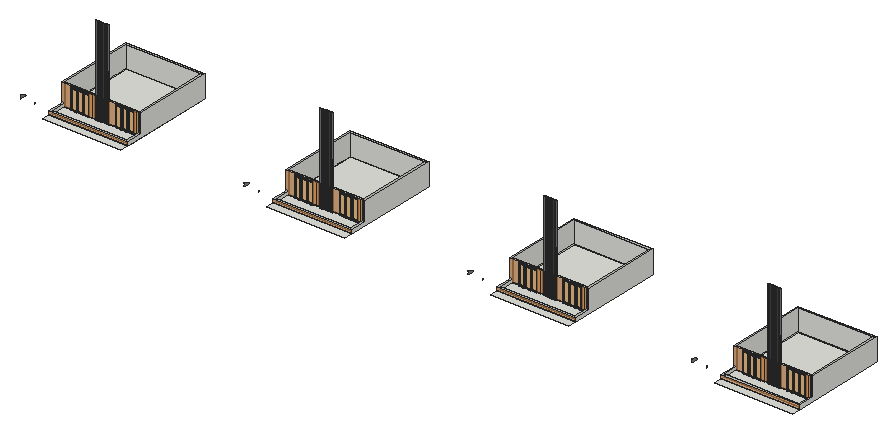
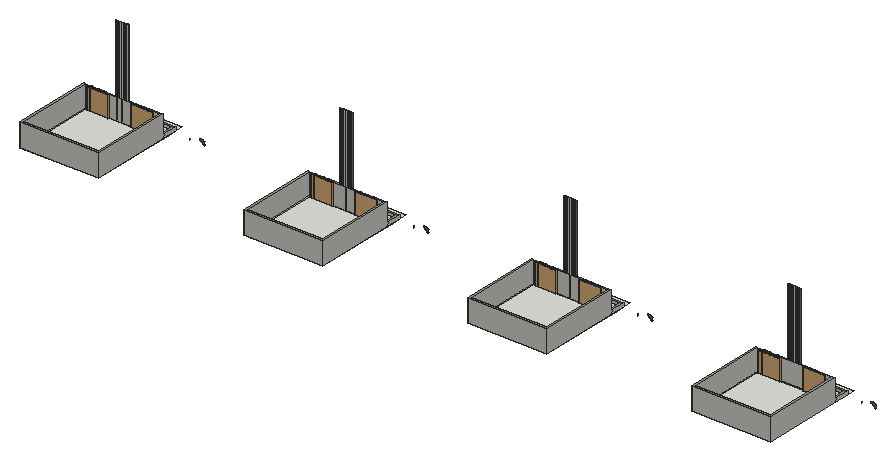
# SketchUp Ruby script. Lengths in inches.
U = 1.inch
M = Sketchup.active_model
def pt(a) = Geom::Point3d.new(a.map { |v| v * U })
def face(e, loops, mat)
  f = e.add_face(loops[0].map { |a| pt(a) })
  loops[1..].each { |l| e.add_face(l.map { |a| pt(a) }).erase! }
  f.material = f.back_material = mat if mat
  f
end
# faces: each face lists its corners as indices into pts; further lists are holes
def faces(e, pts, list, mat = nil) = list.each { |f| face(e, (f[0].is_a?(Array) ? f : [f]).map { |l| l.map { |i| pts[i] } }, mat) }
# xy, xz, yz: faces in a plane at the given z, y or x. An outline is a flat list of corners, or four numbers for a rectangle; further outlines are holes
def ring(l) = l.size == 4 ? [[l[0], l[1]], [l[2], l[1]], [l[2], l[3]], [l[0], l[3]]] : l.each_slice(2).to_a
def flat(e, list, mat, &to3) = list.each { |f| face(e, (f[0].is_a?(Array) ? f : [f]).map { |l| ring(l).map { |u, v| to3.(u, v) } }, mat) }
def xy(e, z, list, mat = nil) = flat(e, list, mat) { |x, y| [x, y, z] }
def xz(e, y, list, mat = nil) = flat(e, list, mat) { |x, z| [x, y, z] }
def yz(e, x, list, mat = nil) = flat(e, list, mat) { |y, z| [x, y, z] }
def lines(e, pts, list) = list.each { |a, b| e.add_line(pt(pts[a]), pt(pts[b])) }
# prism: a flat outline (further loops are holes) pulled along v
def prism(e, loops, v, mat = nil)
  f = face(e, loops, mat); d = Geom::Vector3d.new(v.map { |x| x * U })
  f.pushpull(f.normal.samedirection?(d) ? d.length : -d.length)
end
def box(e, o, s, mat = nil) = prism(e, [[o, [o[0] + s[0], o[1], o[2]], [o[0] + s[0], o[1] + s[1], o[2]], [o[0], o[1] + s[1], o[2]]]], [0, 0, s[2]], mat)
def at(x, y, z, deg = 0) = Geom::Transformation.translation(pt([x, y, z])) * Geom::Transformation.rotation(ORIGIN, Z_AXIS, deg.degrees)
def axes(o, x, y, z) = Geom::Transformation.new([*x, 0, *y, 0, *z, 0, *pt(o).to_a, 1])
def part(name) = M.definitions.add(name)
# library, detail: a bought-in or finely detailed component or shape, given as its bounding box
def library(name, o, s) = part(name).tap { |d| box(d.entities, o, s) }
def detail(e, o, s) = box(e.add_group.entities, o, s)
def put(e, d, t, mat = nil) = e.add_instance(d, t).tap { |i| i.material = mat if mat }
def group(e, t, mat = nil) = e.add_group.tap { |g| g.transformation = t; g.material = mat if mat }.entities
root = M.entities
M.materials.add("Wine2").color = [0, 0, 0]
M.materials["Wine2"].alpha = 0
M.materials.add("[0043_SaddleBrown]4").color = [124, 123, 122]
M.materials.add("[0130_Gainsboro]").color = [39, 45, 50]
M.materials.add("[Granite Dark Gray]").color = [69, 68, 68]
M.materials.add("[Stone Vein Gray]").color = [119, 119, 119]
M.materials.add("[Wood Floor]").color = [224, 152, 88]
M.materials["[Wood Floor]"].alpha = 0.68
c1 = part("Framed glazing panel")
xy(c1.entities,0,[[0,-0.98,43.07,0],[0,0,43.07,1.4]],"[0130_Gainsboro]")
xy(c1.entities,0.3,[[0.3,-1.43,42.77,-0.98]],"[0130_Gainsboro]")
xy(c1.entities,2.95,[[2.95,-1.43,40.12,-0.63],[2.95,-0.63,40.12,0],[2.95,0,40.12,0.64],[2.95,0.64,40.12,1.4]],"[0130_Gainsboro]")
xy(c1.entities,3.54,[[3.54,-0.63,39.53,0],[3.54,0,39.53,0.64]],"[0130_Gainsboro]")
xy(c1.entities,111.8125,[[3.54,-0.63,39.53,0],[3.54,0,39.53,0.64]],"[0130_Gainsboro]")
xy(c1.entities,112.4,[[2.95,-1.43,40.12,-0.63],[2.95,-0.63,40.12,0],[2.95,0,40.12,0.64],[2.95,0.64,40.12,1.4]],"[0130_Gainsboro]")
xy(c1.entities,115.05,[[0.3,-1.43,42.77,-0.98]],"[0130_Gainsboro]")
xy(c1.entities,115.35,[[0,-0.98,43.07,0],[0,0,43.07,1.4]],"[0130_Gainsboro]")
xz(c1.entities,-1.43,[[[0.3,0.3,42.77,115.05],[2.95,2.95,40.12,112.4]]],"[0130_Gainsboro]")
xz(c1.entities,-0.98,[[[0,0,43.07,115.35],[0.3,0.3,42.77,115.05]]],"[0130_Gainsboro]")
xz(c1.entities,-0.63,[[[2.95,2.95,40.12,112.4],[3.54,3.54,39.53,111.8125]]],"[0130_Gainsboro]")
xz(c1.entities,0,[[3.54,3.54,39.53,111.8125]],"Wine2")
xz(c1.entities,0,[[[0,0,43.07,115.35],[2.95,2.95,40.12,112.4]],[[2.95,2.95,40.12,112.4],[3.54,3.54,39.53,111.8125]]],"[0130_Gainsboro]")
xz(c1.entities,0.64,[[[2.95,2.95,40.12,112.4],[3.54,3.54,39.53,111.8125]]],"[0130_Gainsboro]")
xz(c1.entities,1.4,[[[0,0,43.07,115.35],[2.95,2.95,40.12,112.4]]],"[0130_Gainsboro]")
yz(c1.entities,0,[[-0.98,0,0,115.35],[0,0,1.4,115.35]],"[0130_Gainsboro]")
yz(c1.entities,0.3,[[-1.43,0.3,-0.98,115.05]],"[0130_Gainsboro]")
yz(c1.entities,2.95,[[-1.43,2.95,-0.63,112.4],[-0.63,2.95,0,112.4],[0,2.95,0.64,112.4],[0.64,2.95,1.4,112.4]],"[0130_Gainsboro]")
yz(c1.entities,3.54,[[-0.63,3.54,0,111.8125],[0,3.54,0.64,111.8125]],"[0130_Gainsboro]")
yz(c1.entities,39.53,[[-0.63,3.54,0,111.8125],[0,3.54,0.64,111.8125]],"[0130_Gainsboro]")
yz(c1.entities,40.12,[[-1.43,2.95,-0.63,112.4],[-0.63,2.95,0,112.4],[0,2.95,0.64,112.4],[0.64,2.95,1.4,112.4]],"[0130_Gainsboro]")
yz(c1.entities,42.77,[[-1.43,0.3,-0.98,115.05]],"[0130_Gainsboro]")
yz(c1.entities,43.07,[[-0.98,0,0,115.35],[0,0,1.4,115.35]],"[0130_Gainsboro]")
c2 = part("Glazing assembly")
put(c2.entities,c1,axes([90.57,1.43,0],[1.05148,0,0],[0,1,0],[0,0,1]))
put(c2.entities,c1,axes([0,1.43,0],[1.05148,0,0],[0,1,0],[0,0,1]))
put(c2.entities,c1,axes([45.29,1.43,0],[1.05148,0,0],[0,1,0],[0,0,1]))
c3 = library("Curtains",[0,0,0],[121.73,8.19,117.22])
xy(root,268.25,[[563.08,657.03,978.86,1085.17],[1813.71,657.03,2229.49,1085.17],[3064.33,657.03,3480.11,1085.17],[4314.96,657.03,4730.74,1085.17]])
xy(root,268.4375,[[551.76,515.0625,990.19,559.875],[1802.38,515.0625,2240.81,559.875],[3053.01,515.0625,3491.44,559.875],[4303.63,515.0625,4742.06,559.875],[551.76,559.875,990.19,589.17],
  [1802.38,559.875,2240.81,589.17],[3053.01,559.875,3491.44,589.17],[4303.63,559.875,4742.06,589.17],[[551.76,589.17,990.19,1096.5],[835.39,595.44,979.42,595.44,979.42,1090.24,558.02,1090.24,558.02,616,835.39,616]],[[1802.38,589.17,2240.81,1096.5],[2086.01,595.44,2230.05,595.44,2230.05,1090.24,1808.65,1090.24,1808.65,616,2086.01,616]],
  [[3053.01,589.17,3491.44,1096.5],[3336.64,595.44,3480.67,595.44,3480.67,1090.24,3059.27,1090.24,3059.27,616,3336.64,616]],[[4303.63,589.17,4742.06,1096.5],[4587.26,595.44,4731.3,595.44,4731.3,1090.24,4309.9,1090.24,4309.9,616,4587.26,616]]])
xy(root,274.4375,[[563.08,571.2,978.86,571.2,978.86,651.03,951.01,651.03,951.01,657.03,849.76,657.03,849.76,651.03,814.68,651.03,814.68,648.85,805.57,648.85,805.57,651.03,801.81,651.03,801.81,648.85,792.69,648.85,792.69,651.03,789.43,651.03,789.43,648.85,780.32,648.85,780.32,651.03,777.31,651.03,777.31,648.85,768.19,648.85,768.19,651.03,764.56,651.03,764.56,647.91,755.44,647.91,755.44,651.03,751.56,651.03,751.56,647.91,742.44,647.91,742.44,651.03,703.26,651.03,703.26,657.03,602.01,657.03,602.01,651.03,563.08,651.03],[1813.71,571.2,2229.49,571.2,2229.49,651.03,2201.63,651.03,2201.63,657.03,2100.38,657.03,2100.38,651.03,2065.31,651.03,2065.31,648.85,2056.19,648.85,2056.19,651.03,2052.43,651.03,2052.43,648.85,2043.32,648.85,2043.32,651.03,2040.06,651.03,2040.06,648.85,2030.94,648.85,2030.94,651.03,2027.93,651.03,2027.93,648.85,2018.82,648.85,2018.82,651.03,2015.18,651.03,2015.18,647.91,2006.07,647.91,2006.07,651.03,2002.18,651.03,2002.18,647.91,1993.07,647.91,1993.07,651.03,1953.89,651.03,1953.89,657.03,1852.64,657.03,1852.64,651.03,1813.71,651.03],[3064.33,571.2,3480.11,571.2,3480.11,651.03,3452.26,651.03,3452.26,657.03,3351.01,657.03,3351.01,651.03,3315.93,651.03,3315.93,648.85,3306.82,648.85,3306.82,651.03,3303.06,651.03,3303.06,648.85,3293.94,648.85,3293.94,651.03,3290.68,651.03,3290.68,648.85,3281.57,648.85,3281.57,651.03,3278.56,651.03,3278.56,648.85,3269.44,648.85,3269.44,651.03,3265.81,651.03,3265.81,647.91,3256.69,647.91,3256.69,651.03,3252.81,651.03,3252.81,647.91,3243.69,647.91,3243.69,651.03,3204.51,651.03,3204.51,657.03,3103.26,657.03,3103.26,651.03,3064.33,651.03],[4314.96,571.2,4730.74,571.2,4730.74,651.03,4702.88,651.03,4702.88,657.03,4601.63,657.03,4601.63,651.03,4566.56,651.03,4566.56,648.85,4557.44,648.85,4557.44,651.03,4553.68,651.03,4553.68,648.85,4544.57,648.85,4544.57,651.03,4541.31,651.03,4541.31,648.85,4532.19,648.85,4532.19,651.03,4529.18,651.03,4529.18,648.85,4520.07,648.85,4520.07,651.03,4516.43,651.03,4516.43,647.91,4507.32,647.91,4507.32,651.03,4503.43,651.03,4503.43,647.91,4494.32,647.91,4494.32,651.03,4455.14,651.03,4455.14,657.03,4353.89,657.03,4353.89,651.03,4314.96,651.03],[563.08,657.03,978.86,1085.17],
  [1813.71,657.03,2229.49,1085.17],[3064.33,657.03,3480.11,1085.17],[4314.96,657.03,4730.74,1085.17]])
xz(root,559.875,[[551.76,268.4375,990.19,289.5625],[1802.38,268.4375,2240.81,289.5625],[3053.01,268.4375,3491.44,289.5625],[4303.63,268.4375,4742.06,289.5625]],"[Wood Floor]")
xz(root,571.2,[[563.08,274.4375,978.86,289.5625],[1813.71,274.4375,2229.49,289.5625],[3064.33,274.4375,3480.11,289.5625],[4314.96,274.4375,4730.74,289.5625]])
xz(root,589.17,[[448.37,274.24,448.14,274.83,447.96,275.43,447.8125,276.04,447.71,276.65,447.65,277.26,447.625,277.875,447.65,278.49,447.71,279.11,447.8125,279.72,447.96,280.32,448.14,280.92,448.37,281.52],[1698.99,274.24,1698.77,274.83,1698.58,275.43,1698.4375,276.04,1698.33,276.65,1698.27,277.26,1698.25,277.875,1698.27,278.49,1698.33,279.11,1698.4375,279.72,1698.58,280.32,1698.77,280.92,1698.99,281.52],[2949.62,274.24,2949.39,274.83,2949.21,275.43,2949.0625,276.04,2948.96,276.65,2948.9,277.26,2948.875,277.875,2948.9,278.49,2948.96,279.11,2949.0625,279.72,2949.21,280.32,2949.39,280.92,2949.62,281.52],[4200.24,274.24,4200.02,274.83,4199.83,275.43,4199.6875,276.04,4199.58,276.65,4199.52,277.26,4199.5,277.875,4199.52,278.49,4199.58,279.11,4199.6875,279.72,4199.83,280.32,4200.02,280.92,4200.24,281.52],[367.98,274.88,367.98,278.09,368.99,279,369.85,279.99,370.53,281.06,371.02,282.17,371.32,283.32,371.42,284.48,371.32,285.65,371.02,286.8,370.53,287.91,369.85,288.98,368.99,289.97,367.98,290.875,367.98,291.93,369.26,292.12,370.53,292.36,371.79,292.65,373.02,292.98,374.22,293.37,375.39,293.79,376.54,294.26,377.64,294.77,378.71,295.33,379.74,295.92,380.72,296.55,381.65,297.22,382.38,297.73,383.16,298.2,383.98,298.63,384.84,299.02,385.74,299.36,386.67,299.65,387.625,299.9,388.6,300.09,389.6,300.24,390.61,300.33,391.62,300.37,392.64,300.36,393.45,300.26,394.22,300.04,394.89,299.69,395.4375,299.24,395.83,298.72,396.06,298.15,396.09,297.55,395.95,296.97,395.62,296.42,395.13,295.94,394.5,295.55,393.77,295.28,393.66,295.875,393.34,296.43,392.83,296.91,392.17,297.28,391.4,297.51,390.57,297.58,389.74,297.51,388.97,297.28,388.3,296.91,387.79,296.43,387.47,295.875,387.36,295.28,387.32,294.8,387.29,294.33,387.29,293.85,387.3,293.375,387.32,292.9,387.37,292.43,387.43,291.95,387.51,291.48,387.61,291.01,387.72,290.54,387.85,290.08,388,289.61,386.54,289.1875,385.13,288.68,383.78,288.1,382.49,287.43,381.29,286.7,380.17,285.9,379.14,285.04,378.2,284.12,377.375,283.15,376.66,282.14,376.05,281.09,375.57,280.01,375.04,279.51,374.5,279.02,373.93,278.54,373.34,278.07,372.73,277.625,372.11,277.1875,371.46,276.76,370.8,276.36,370.12,275.97,369.42,275.59,368.7,275.23],
  [1618.6,274.88,1618.6,278.09,1619.62,279,1620.48,279.99,1621.16,281.06,1621.65,282.17,1621.95,283.32,1622.05,284.48,1621.95,285.65,1621.65,286.8,1621.16,287.91,1620.48,288.98,1619.62,289.97,1618.6,290.875,1618.6,291.93,1619.89,292.12,1621.16,292.36,1622.41,292.65,1623.64,292.98,1624.85,293.37,1626.02,293.79,1627.16,294.26,1628.27,294.77,1629.33,295.33,1630.36,295.92,1631.34,296.55,1632.28,297.22,1633,297.73,1633.78,298.2,1634.6,298.63,1635.47,299.02,1636.36,299.36,1637.29,299.65,1638.25,299.9,1639.23,300.09,1640.23,300.24,1641.23,300.33,1642.25,300.37,1643.26,300.36,1644.08,300.26,1644.84,300.04,1645.52,299.69,1646.0625,299.24,1646.46,298.72,1646.68,298.15,1646.72,297.55,1646.57,296.97,1646.24,296.42,1645.75,295.94,1645.125,295.55,1644.39,295.28,1644.28,295.875,1643.96,296.43,1643.46,296.91,1642.79,297.28,1642.02,297.51,1641.19,297.58,1640.36,297.51,1639.59,297.28,1638.93,296.91,1638.42,296.43,1638.1,295.875,1637.99,295.28,1637.95,294.8,1637.92,294.33,1637.91,293.85,1637.92,293.375,1637.95,292.9,1637.99,292.43,1638.05,291.95,1638.13,291.48,1638.23,291.01,1638.35,290.54,1638.48,290.08,1638.63,289.61,1637.17,289.1875,1635.75,288.68,1634.4,288.1,1633.12,287.43,1631.91,286.7,1630.79,285.9,1629.76,285.04,1628.83,284.12,1628,283.15,1627.28,282.14,1626.68,281.09,1626.19,280.01,1625.67,279.51,1625.12,279.02,1624.55,278.54,1623.97,278.07,1623.36,277.625,1622.73,277.1875,1622.09,276.76,1621.42,276.36,1620.74,275.97,1620.04,275.59,1619.33,275.23],[2869.23,274.88,2869.23,278.09,2870.24,279,2871.1,279.99,2871.78,281.06,2872.27,282.17,2872.57,283.32,2872.67,284.48,2872.57,285.65,2872.27,286.8,2871.78,287.91,2871.1,288.98,2870.24,289.97,2869.23,290.875,2869.23,291.93,2870.51,292.12,2871.78,292.36,2873.04,292.65,2874.27,292.98,2875.47,293.37,2876.64,293.79,2877.79,294.26,2878.89,294.77,2879.96,295.33,2880.99,295.92,2881.97,296.55,2882.9,297.22,2883.63,297.73,2884.41,298.2,2885.23,298.63,2886.09,299.02,2886.99,299.36,2887.92,299.65,2888.875,299.9,2889.85,300.09,2890.85,300.24,2891.86,300.33,2892.87,300.37,2893.89,300.36,2894.7,300.26,2895.47,300.04,2896.14,299.69,2896.6875,299.24,2897.08,298.72,2897.31,298.15,2897.34,297.55,2897.2,296.97,2896.87,296.42,2896.38,295.94,2895.75,295.55,2895.02,295.28,2894.91,295.875,2894.59,296.43,2894.08,296.91,2893.42,297.28,2892.65,297.51,2891.82,297.58,2890.99,297.51,2890.22,297.28,2889.55,296.91,2889.04,296.43,2888.72,295.875,2888.61,295.28,2888.57,294.8,2888.54,294.33,2888.54,293.85,2888.55,293.375,2888.57,292.9,2888.62,292.43,2888.68,291.95,2888.76,291.48,2888.86,291.01,2888.97,290.54,2889.1,290.08,2889.25,289.61,2887.79,289.1875,2886.38,288.68,2885.03,288.1,2883.74,287.43,2882.54,286.7,2881.42,285.9,2880.39,285.04,2879.45,284.12,2878.625,283.15,2877.91,282.14,2877.3,281.09,2876.82,280.01,2876.29,279.51,2875.75,279.02,2875.18,278.54,2874.59,278.07,2873.98,277.625,2873.36,277.1875,2872.71,276.76,2872.05,276.36,2871.37,275.97,2870.67,275.59,2869.95,275.23],[4119.85,274.88,4119.85,278.09,4120.87,279,4121.73,279.99,4122.41,281.06,4122.9,282.17,4123.2,283.32,4123.3,284.48,4123.2,285.65,4122.9,286.8,4122.41,287.91,4121.73,288.98,4120.87,289.97,4119.85,290.875,4119.85,291.93,4121.14,292.12,4122.41,292.36,4123.66,292.65,4124.89,292.98,4126.1,293.37,4127.27,293.79,4128.41,294.26,4129.52,294.77,4130.58,295.33,4131.61,295.92,4132.59,296.55,4133.53,297.22,4134.25,297.73,4135.03,298.2,4135.85,298.63,4136.72,299.02,4137.61,299.36,4138.54,299.65,4139.5,299.9,4140.48,300.09,4141.48,300.24,4142.48,300.33,4143.5,300.37,4144.51,300.36,4145.33,300.26,4146.09,300.04,4146.77,299.69,4147.3125,299.24,4147.71,298.72,4147.93,298.15,4147.97,297.55,4147.82,296.97,4147.49,296.42,4147,295.94,4146.375,295.55,4145.64,295.28,4145.53,295.875,4145.21,296.43,4144.71,296.91,4144.04,297.28,4143.27,297.51,4142.44,297.58,4141.61,297.51,4140.84,297.28,4140.18,296.91,4139.67,296.43,4139.35,295.875,4139.24,295.28,4139.2,294.8,4139.17,294.33,4139.16,293.85,4139.17,293.375,4139.2,292.9,4139.24,292.43,4139.3,291.95,4139.38,291.48,4139.48,291.01,4139.6,290.54,4139.73,290.08,4139.88,289.61,4138.42,289.1875,4137,288.68,4135.65,288.1,4134.37,287.43,4133.16,286.7,4132.04,285.9,4131.01,285.04,4130.08,284.12,4129.25,283.15,4128.53,282.14,4127.93,281.09,4127.44,280.01,4126.92,279.51,4126.37,279.02,4125.8,278.54,4125.22,278.07,4124.61,277.625,4123.98,277.1875,4123.34,276.76,4122.67,276.36,4121.99,275.97,4121.29,275.59,4120.58,275.23]],"[0043_SaddleBrown]4")
xz(root,647.91,[[755.44,274.4375,764.56,771.4375],[2006.07,274.4375,2015.18,771.4375],[3256.69,274.4375,3265.81,771.4375],[4507.32,274.4375,4516.43,771.4375]],"[Granite Dark Gray]")
xz(root,647.91,[[742.44,274.4375,751.56,274.4375,751.56,771.4375,742.44,771.4375,742.44,665.9375,744.19,665.9375,744.19,662.4375,742.44,662.4375,742.44,541.1875,744.19,541.1875,744.19,538.1875,742.44,538.1875,742.44,413.5,744.38,413.5,744.38,410.625,742.44,410.625],[1993.07,274.4375,2002.18,274.4375,2002.18,771.4375,1993.07,771.4375,1993.07,665.9375,1994.82,665.9375,1994.82,662.4375,1993.07,662.4375,1993.07,541.1875,1994.82,541.1875,1994.82,538.1875,1993.07,538.1875,1993.07,413.5,1995.01,413.5,1995.01,410.625,1993.07,410.625],[3243.69,274.4375,3252.81,274.4375,3252.81,771.4375,3243.69,771.4375,3243.69,665.9375,3245.44,665.9375,3245.44,662.4375,3243.69,662.4375,3243.69,541.1875,3245.44,541.1875,3245.44,538.1875,3243.69,538.1875,3243.69,413.5,3245.63,413.5,3245.63,410.625,3243.69,410.625],[4494.32,274.4375,4503.43,274.4375,4503.43,771.4375,4494.32,771.4375,4494.32,665.9375,4496.07,665.9375,4496.07,662.4375,4494.32,662.4375,4494.32,541.1875,4496.07,541.1875,4496.07,538.1875,4494.32,538.1875,4494.32,413.5,4496.26,413.5,4496.26,410.625,4494.32,410.625]],"[Stone Vein Gray]")
xz(root,648.85,[[768.19,274.4375,777.31,771.4375],[780.32,274.4375,789.43,771.4375],[792.69,274.4375,801.81,771.4375],[2018.82,274.4375,2027.93,771.4375],[2030.94,274.4375,2040.06,771.4375],
  [2043.32,274.4375,2052.43,771.4375],[3269.44,274.4375,3278.56,771.4375],[3281.57,274.4375,3290.68,771.4375],[3293.94,274.4375,3303.06,771.4375],[4520.07,274.4375,4529.18,771.4375],
  [4532.19,274.4375,4541.31,771.4375],[4544.57,274.4375,4553.68,771.4375]],"[Granite Dark Gray]")
xz(root,648.85,[[805.57,274.4375,814.68,274.4375,814.68,662.4375,812.81,662.4375,812.81,665.9375,814.68,665.9375,814.68,771.4375,805.57,771.4375],[2056.19,274.4375,2065.31,274.4375,2065.31,662.4375,2063.43,662.4375,2063.43,665.9375,2065.31,665.9375,2065.31,771.4375,2056.19,771.4375],[3306.82,274.4375,3315.93,274.4375,3315.93,662.4375,3314.06,662.4375,3314.06,665.9375,3315.93,665.9375,3315.93,771.4375,3306.82,771.4375],[4557.44,274.4375,4566.56,274.4375,4566.56,662.4375,4564.68,662.4375,4564.68,665.9375,4566.56,665.9375,4566.56,771.4375,4557.44,771.4375]],"[Stone Vein Gray]")
xz(root,651.03,[[814.68,274.4375,814.89,410.625],[2065.31,274.4375,2065.52,410.625],[3315.93,274.4375,3316.14,410.625],[4566.56,274.4375,4566.77,410.625]])
xz(root,651.03,[[764.56,274.4375,768.19,771.4375],[777.31,274.4375,780.32,771.4375],[789.43,274.4375,792.69,771.4375],[2015.18,274.4375,2018.82,771.4375],[2027.93,274.4375,2030.94,771.4375],
  [2040.06,274.4375,2043.32,771.4375],[3265.81,274.4375,3269.44,771.4375],[3278.56,274.4375,3281.57,771.4375],[3290.68,274.4375,3293.94,771.4375],[4516.43,274.4375,4520.07,771.4375],
  [4529.18,274.4375,4532.19,771.4375],[4541.31,274.4375,4544.57,771.4375]],"[Granite Dark Gray]")
xz(root,651.03,[[751.56,274.4375,755.44,771.4375],[801.81,274.4375,805.57,771.4375],[2002.18,274.4375,2006.07,771.4375],[2052.43,274.4375,2056.19,771.4375],[3252.81,274.4375,3256.69,771.4375],
  [3303.06,274.4375,3306.82,771.4375],[4503.43,274.4375,4507.32,771.4375],[4553.68,274.4375,4557.44,771.4375]],"[Stone Vein Gray]")
xz(root,651.03,[[563.08,274.4375,602.01,274.4375,602.01,388.875,703.26,388.875,703.26,274.4375,742.44,274.4375,742.44,394.4375,551.76,394.4375,551.76,293,563.08,293],[814.89,274.4375,849.76,274.4375,849.76,388.875,951.01,388.875,951.01,274.4375,978.86,274.4375,978.86,394.4375,814.89,394.4375],[1813.71,274.4375,1852.64,274.4375,1852.64,388.875,1953.89,388.875,1953.89,274.4375,1993.07,274.4375,1993.07,394.4375,1802.38,394.4375,1802.38,293,1813.71,293],[2065.52,274.4375,2100.38,274.4375,2100.38,388.875,2201.63,388.875,2201.63,274.4375,2229.49,274.4375,2229.49,394.4375,2065.52,394.4375],[3064.33,274.4375,3103.26,274.4375,3103.26,388.875,3204.51,388.875,3204.51,274.4375,3243.69,274.4375,3243.69,394.4375,3053.01,394.4375,3053.01,293,3064.33,293],
  [3316.14,274.4375,3351.01,274.4375,3351.01,388.875,3452.26,388.875,3452.26,274.4375,3480.11,274.4375,3480.11,394.4375,3316.14,394.4375],[4314.96,274.4375,4353.89,274.4375,4353.89,388.875,4455.14,388.875,4455.14,274.4375,4494.32,274.4375,4494.32,394.4375,4303.63,394.4375,4303.63,293,4314.96,293],[4566.77,274.4375,4601.63,274.4375,4601.63,388.875,4702.88,388.875,4702.88,274.4375,4730.74,274.4375,4730.74,394.4375,4566.77,394.4375]],"[Wood Floor]")
xz(root,657.03,[[563.08,268.25,602.01,274.4375],[602.01,268.25,703.26,274.4375],[703.26,268.25,849.76,274.4375],[849.76,268.25,951.01,274.4375],[951.01,268.25,978.86,274.4375],
  [1813.71,268.25,1852.64,274.4375],[1852.64,268.25,1953.89,274.4375],[1953.89,268.25,2100.38,274.4375],[2100.38,268.25,2201.63,274.4375],[2201.63,268.25,2229.49,274.4375],
  [3064.33,268.25,3103.26,274.4375],[3103.26,268.25,3204.51,274.4375],[3204.51,268.25,3351.01,274.4375],[3351.01,268.25,3452.26,274.4375],[3452.26,268.25,3480.11,274.4375],
  [4314.96,268.25,4353.89,274.4375],[4353.89,268.25,4455.14,274.4375],[4455.14,268.25,4601.63,274.4375],[4601.63,268.25,4702.88,274.4375],[4702.88,268.25,4730.74,274.4375],
  [563.08,274.4375,563.08,394.4375,978.86,394.4375,978.86,274.4375,951.01,274.4375,951.01,388.875,849.76,388.875,849.76,274.4375,703.26,274.4375,703.26,388.875,602.01,388.875,602.01,274.4375],[1813.71,274.4375,1813.71,394.4375,2229.49,394.4375,2229.49,274.4375,2201.63,274.4375,2201.63,388.875,2100.38,388.875,2100.38,274.4375,1953.89,274.4375,1953.89,388.875,1852.64,388.875,1852.64,274.4375],[3064.33,274.4375,3064.33,394.4375,3480.11,394.4375,3480.11,274.4375,3452.26,274.4375,3452.26,388.875,3351.01,388.875,3351.01,274.4375,3204.51,274.4375,3204.51,388.875,3103.26,388.875,3103.26,274.4375],[4314.96,274.4375,4314.96,394.4375,4730.74,394.4375,4730.74,274.4375,4702.88,274.4375,4702.88,388.875,4601.63,388.875,4601.63,274.4375,4455.14,274.4375,4455.14,388.875,4353.89,388.875,4353.89,274.4375]])
xz(root,1085.17,[[563.08,268.25,978.86,274.4375],[1813.71,268.25,2229.49,274.4375],[3064.33,268.25,3480.11,274.4375],[4314.96,268.25,4730.74,274.4375],[563.08,274.4375,978.86,394.4375],
  [1813.71,274.4375,2229.49,394.4375],[3064.33,274.4375,3480.11,394.4375],[4314.96,274.4375,4730.74,394.4375]])
xz(root,1096.5,[[551.76,268.4375,990.19,394.4375],[1802.38,268.4375,2240.81,394.4375],[3053.01,268.4375,3491.44,394.4375],[4303.63,268.4375,4742.06,394.4375]])
yz(root,551.76,[[559.875,268.4375,640.11,289.5625],[640.11,268.4375,640.11,289.5625,651.03,289.5625,651.03,394.4375,1096.5,394.4375,1096.5,268.4375]])
yz(root,563.08,[[657.03,268.25,1085.17,274.4375],[571.2,274.4375,651.03,289.5625],[657.03,274.4375,1085.17,394.4375]])
yz(root,602.01,[[651.03,274.4375,657.03,388.875]])
yz(root,703.26,[[651.03,274.4375,657.03,388.875]])
yz(root,742.44,[[647.91,274.4375,651.03,394.4375]])
yz(root,751.56,[[647.91,274.4375,651.03,771.4375]])
yz(root,755.44,[[647.91,274.4375,651.03,394.4375]])
yz(root,764.56,[[647.91,274.4375,651.03,771.4375]])
yz(root,768.19,[[648.85,274.4375,651.03,394.4375]])
yz(root,777.31,[[648.85,274.4375,651.03,771.4375]])
yz(root,780.32,[[648.85,274.4375,651.03,394.4375]])
yz(root,789.43,[[648.85,274.4375,651.03,771.4375]])
yz(root,792.69,[[648.85,274.4375,651.03,394.4375]])
yz(root,801.81,[[648.85,274.4375,651.03,771.4375]])
yz(root,805.57,[[648.85,274.4375,651.03,394.4375]])
yz(root,814.68,[[648.85,274.4375,651.03,538.1875]])
yz(root,849.76,[[651.03,274.4375,657.03,388.875]])
yz(root,951.01,[[651.03,274.4375,657.03,388.875]])
yz(root,978.86,[[657.03,268.25,1085.17,274.4375],[571.2,274.4375,651.03,289.5625],[657.03,274.4375,1085.17,394.4375]])
yz(root,990.19,[[559.875,268.4375,1096.5,268.4375,1096.5,394.4375,651.03,394.4375,651.03,289.5625,559.875,289.5625]])
yz(root,1802.38,[[559.875,268.4375,640.11,289.5625],[640.11,268.4375,640.11,289.5625,651.03,289.5625,651.03,394.4375,1096.5,394.4375,1096.5,268.4375]])
yz(root,1813.71,[[657.03,268.25,1085.17,274.4375],[571.2,274.4375,651.03,289.5625],[657.03,274.4375,1085.17,394.4375]])
yz(root,1852.64,[[651.03,274.4375,657.03,388.875]])
yz(root,1953.89,[[651.03,274.4375,657.03,388.875]])
yz(root,1993.07,[[647.91,274.4375,651.03,394.4375]])
yz(root,2002.18,[[647.91,274.4375,651.03,771.4375]])
yz(root,2006.07,[[647.91,274.4375,651.03,394.4375]])
yz(root,2015.18,[[647.91,274.4375,651.03,771.4375]])
yz(root,2018.82,[[648.85,274.4375,651.03,394.4375]])
yz(root,2027.93,[[648.85,274.4375,651.03,771.4375]])
yz(root,2030.94,[[648.85,274.4375,651.03,394.4375]])
yz(root,2040.06,[[648.85,274.4375,651.03,771.4375]])
yz(root,2043.32,[[648.85,274.4375,651.03,394.4375]])
yz(root,2052.43,[[648.85,274.4375,651.03,771.4375]])
yz(root,2056.19,[[648.85,274.4375,651.03,394.4375]])
yz(root,2065.31,[[648.85,274.4375,651.03,538.1875]])
yz(root,2100.38,[[651.03,274.4375,657.03,388.875]])
yz(root,2201.63,[[651.03,274.4375,657.03,388.875]])
yz(root,2229.49,[[657.03,268.25,1085.17,274.4375],[571.2,274.4375,651.03,289.5625],[657.03,274.4375,1085.17,394.4375]])
yz(root,2240.81,[[559.875,268.4375,1096.5,268.4375,1096.5,394.4375,651.03,394.4375,651.03,289.5625,559.875,289.5625]])
yz(root,3053.01,[[559.875,268.4375,640.11,289.5625],[640.11,268.4375,640.11,289.5625,651.03,289.5625,651.03,394.4375,1096.5,394.4375,1096.5,268.4375]])
yz(root,3064.33,[[657.03,268.25,1085.17,274.4375],[571.2,274.4375,651.03,289.5625],[657.03,274.4375,1085.17,394.4375]])
yz(root,3103.26,[[651.03,274.4375,657.03,388.875]])
yz(root,3204.51,[[651.03,274.4375,657.03,388.875]])
yz(root,3243.69,[[647.91,274.4375,651.03,394.4375]])
yz(root,3252.81,[[647.91,274.4375,651.03,771.4375]])
yz(root,3256.69,[[647.91,274.4375,651.03,394.4375]])
yz(root,3265.81,[[647.91,274.4375,651.03,771.4375]])
yz(root,3269.44,[[648.85,274.4375,651.03,394.4375]])
yz(root,3278.56,[[648.85,274.4375,651.03,771.4375]])
yz(root,3281.57,[[648.85,274.4375,651.03,394.4375]])
yz(root,3290.68,[[648.85,274.4375,651.03,771.4375]])
yz(root,3293.94,[[648.85,274.4375,651.03,394.4375]])
yz(root,3303.06,[[648.85,274.4375,651.03,771.4375]])
yz(root,3306.82,[[648.85,274.4375,651.03,394.4375]])
yz(root,3315.93,[[648.85,274.4375,651.03,538.1875]])
yz(root,3351.01,[[651.03,274.4375,657.03,388.875]])
yz(root,3452.26,[[651.03,274.4375,657.03,388.875]])
yz(root,3480.11,[[657.03,268.25,1085.17,274.4375],[571.2,274.4375,651.03,289.5625],[657.03,274.4375,1085.17,394.4375]])
yz(root,3491.44,[[559.875,268.4375,1096.5,268.4375,1096.5,394.4375,651.03,394.4375,651.03,289.5625,559.875,289.5625]])
yz(root,4303.63,[[559.875,268.4375,640.11,289.5625],[640.11,268.4375,640.11,289.5625,651.03,289.5625,651.03,394.4375,1096.5,394.4375,1096.5,268.4375]])
yz(root,4314.96,[[657.03,268.25,1085.17,274.4375],[571.2,274.4375,651.03,289.5625],[657.03,274.4375,1085.17,394.4375]])
yz(root,4353.89,[[651.03,274.4375,657.03,388.875]])
yz(root,4455.14,[[651.03,274.4375,657.03,388.875]])
yz(root,4494.32,[[647.91,274.4375,651.03,394.4375]])
yz(root,4503.43,[[647.91,274.4375,651.03,771.4375]])
yz(root,4507.32,[[647.91,274.4375,651.03,394.4375]])
yz(root,4516.43,[[647.91,274.4375,651.03,771.4375]])
yz(root,4520.07,[[648.85,274.4375,651.03,394.4375]])
yz(root,4529.18,[[648.85,274.4375,651.03,771.4375]])
yz(root,4532.19,[[648.85,274.4375,651.03,394.4375]])
yz(root,4541.31,[[648.85,274.4375,651.03,771.4375]])
yz(root,4544.57,[[648.85,274.4375,651.03,394.4375]])
yz(root,4553.68,[[648.85,274.4375,651.03,771.4375]])
yz(root,4557.44,[[648.85,274.4375,651.03,394.4375]])
yz(root,4566.56,[[648.85,274.4375,651.03,538.1875]])
yz(root,4601.63,[[651.03,274.4375,657.03,388.875]])
yz(root,4702.88,[[651.03,274.4375,657.03,388.875]])
yz(root,4730.74,[[657.03,268.25,1085.17,274.4375],[571.2,274.4375,651.03,289.5625],[657.03,274.4375,1085.17,394.4375]])
yz(root,4742.06,[[559.875,268.4375,1096.5,268.4375,1096.5,394.4375,651.03,394.4375,651.03,289.5625,559.875,289.5625]])
put(root,c2,axes([3102.62,648.91,271.48],[0.75,0,0],[0,0.75,0],[0,0,1.01765]))
put(root,c2,axes([4353.24,648.91,271.48],[0.75,0,0],[0,0.75,0],[0,0,1.01765]))
put(root,c2,axes([601.37,648.91,271.48],[0.75,0,0],[0,0.75,0],[0,0,1.01765]))
put(root,c2,axes([1851.99,648.91,271.48],[0.75,0,0],[0,0.75,0],[0,0,1.01765]))
put(root,c3,at(3102.07,651.68,271.95))
put(root,c3,at(3349.95,651.68,271.95))
put(root,c3,at(4600.57,651.68,271.95))
put(root,c3,at(4352.7,651.68,271.95))
put(root,c3,at(848.7,651.68,271.95))
put(root,c3,at(600.82,651.68,271.95))
put(root,c3,at(1851.45,651.68,271.95))
put(root,c3,at(2099.32,651.68,271.95))
put(root,c2,axes([3352.6875,649.48,274.49],[0.75,0,0],[0,0.75,0],[0,0,1.01765]))
put(root,c2,axes([4603.3125,649.48,274.49],[0.75,0,0],[0,0.75,0],[0,0,1.01765]))
put(root,c2,axes([851.4375,649.48,274.49],[0.75,0,0],[0,0.75,0],[0,0,1.01765]))
put(root,c2,axes([2102.0625,649.48,274.49],[0.75,0,0],[0,0.75,0],[0,0,1.01765]))
